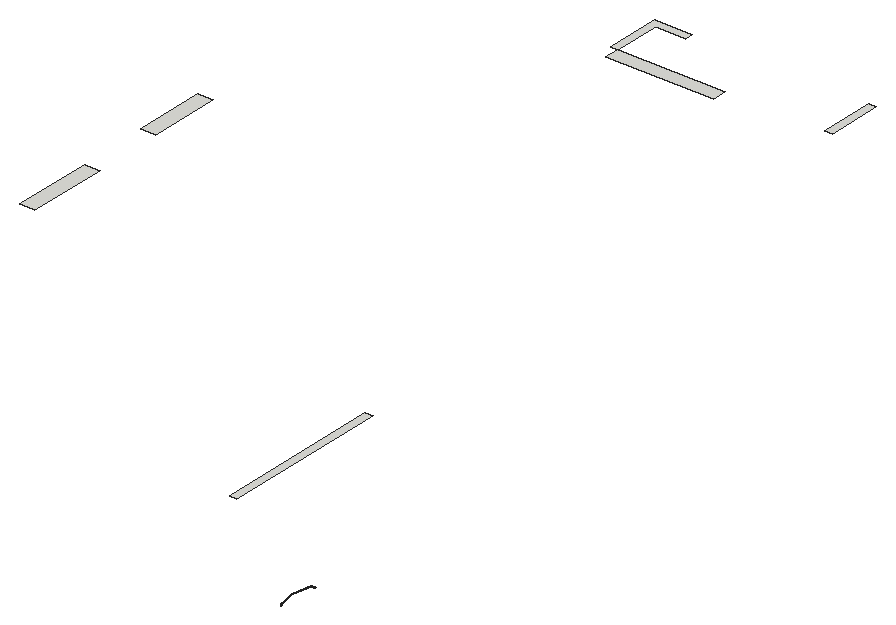
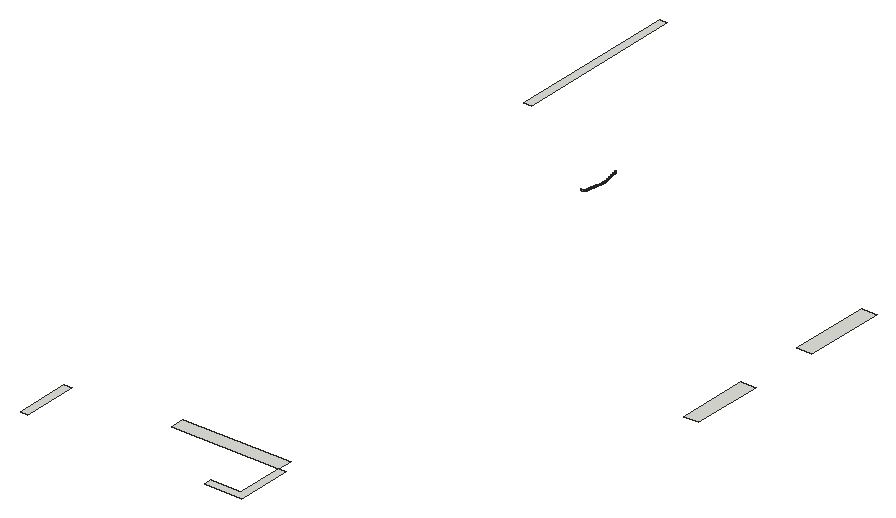
# SketchUp Ruby script. Lengths in inches.
U = 1.inch
M = Sketchup.active_model
def pt(a) = Geom::Point3d.new(a.map { |v| v * U })
def face(e, loops, mat)
  f = e.add_face(loops[0].map { |a| pt(a) })
  loops[1..].each { |l| e.add_face(l.map { |a| pt(a) }).erase! }
  f.material = f.back_material = mat if mat
  f
end
# faces: each face lists its corners as indices into pts; further lists are holes
def faces(e, pts, list, mat = nil) = list.each { |f| face(e, (f[0].is_a?(Array) ? f : [f]).map { |l| l.map { |i| pts[i] } }, mat) }
# xy, xz, yz: faces in a plane at the given z, y or x. An outline is a flat list of corners, or four numbers for a rectangle; further outlines are holes
def ring(l) = l.size == 4 ? [[l[0], l[1]], [l[2], l[1]], [l[2], l[3]], [l[0], l[3]]] : l.each_slice(2).to_a
def flat(e, list, mat, &to3) = list.each { |f| face(e, (f[0].is_a?(Array) ? f : [f]).map { |l| ring(l).map { |u, v| to3.(u, v) } }, mat) }
def xy(e, z, list, mat = nil) = flat(e, list, mat) { |x, y| [x, y, z] }
def xz(e, y, list, mat = nil) = flat(e, list, mat) { |x, z| [x, y, z] }
def yz(e, x, list, mat = nil) = flat(e, list, mat) { |y, z| [x, y, z] }
def lines(e, pts, list) = list.each { |a, b| e.add_line(pt(pts[a]), pt(pts[b])) }
# prism: a flat outline (further loops are holes) pulled along v
def prism(e, loops, v, mat = nil)
  f = face(e, loops, mat); d = Geom::Vector3d.new(v.map { |x| x * U })
  f.pushpull(f.normal.samedirection?(d) ? d.length : -d.length)
end
def box(e, o, s, mat = nil) = prism(e, [[o, [o[0] + s[0], o[1], o[2]], [o[0] + s[0], o[1] + s[1], o[2]], [o[0], o[1] + s[1], o[2]]]], [0, 0, s[2]], mat)
def at(x, y, z, deg = 0) = Geom::Transformation.translation(pt([x, y, z])) * Geom::Transformation.rotation(ORIGIN, Z_AXIS, deg.degrees)
def axes(o, x, y, z) = Geom::Transformation.new([*x, 0, *y, 0, *z, 0, *pt(o).to_a, 1])
def part(name) = M.definitions.add(name)
# library, detail: a bought-in or finely detailed component or shape, given as its bounding box
def library(name, o, s) = part(name).tap { |d| box(d.entities, o, s) }
def detail(e, o, s) = box(e.add_group.entities, o, s)
def put(e, d, t, mat = nil) = e.add_instance(d, t).tap { |i| i.material = mat if mat }
def group(e, t, mat = nil) = e.add_group.tap { |g| g.transformation = t; g.material = mat if mat }.entities
root = M.entities
xy(root,108,[[322.5,47.86,327,149.86],[71,204.86,80,253.05],[198,486.86,262.5,495.62],[193.5,495.875,198,495.875,198,524.36,216.18,524.36,216.18,528.86,193.5,528.86],[322.5,495.875,327,528.86]])
xy(root,108.57,[[71,295.7,80,338.36]])
p = [[329.39,77.66,38.26],[329.36,77.63,38.17],[329.28,77.71,38.17],[329.31,77.74,38.26],[329.48,77.59,38.26],[329.46,77.55,38.17],
  [329.2,77.8,38.17],[329.23,77.82,38.26],[329.13,77.9,38.17],[329.17,77.92,38.26],[329.08,78,38.17],[329.12,78.02,38.26],
  [329.04,78.11,38.17],[329.07,78.125,38.26],[329,78.23,38.17],[329.04,78.24,38.26],[328.96,78.42,38.17],[329,78.43,38.26],
  [328.93,78.61,38.17],[328.97,78.62,38.26],[328.9,78.81,38.17],[328.9375,78.8125,38.26],[328.87,79,38.17],[328.91,79.01,38.26],
  [328.85,79.2,38.17],[328.89,79.2,38.26],[328.83,79.39,38.17],[328.87,79.4,38.26],[328.82,79.59,38.17],[328.86,79.59,38.26],
  [328.8125,79.78,38.17],[328.85,79.79,38.26],[328.8125,79.98,38.17],[328.85,79.98,38.26],[328.8125,80.18,38.17],[328.85,80.18,38.26],
  [328.82,80.375,38.17],[328.86,80.37,38.26],[328.83,80.59,38.17],[328.875,80.59,38.26],[328.61,81.3,38.17],[328.65,81.31,38.26],
  [328.4,81.99,38.17],[328.44,82,38.26],[328.21,82.6875,38.17],[328.25,82.7,38.26],[328.03,83.39,38.17],[328.07,83.4,38.26],
  [327.87,84.09,38.17],[327.91,84.1,38.26],[327.72,84.8,38.17],[327.75,84.8125,38.26],[327.58,85.51,38.17],[327.62,85.52,38.26],
  [327.45,86.23,38.17],[327.49,86.23,38.26],[327.34,86.94,38.17],[327.38,86.95,38.26],[327.24,87.66,38.17],[327.28,87.67,38.26],
  [327.16,88.38,38.17],[327.2,88.38,38.26],[327.09,89.09,38.17],[327.13,89.09,38.26],[327.16,89.81,38.17],[327.2,89.8,38.26],
  [327.24,90.53,38.17],[327.28,90.52,38.26],[327.34,91.24,38.17],[327.38,91.24,38.26],[327.45,91.96,38.17],[327.49,91.95,38.26],
  [327.58,92.67,38.17],[327.62,92.66,38.26],[327.72,93.38,38.17],[327.75,93.375,38.26],[327.87,94.09,38.17],[327.91,94.08,38.26],
  [328.03,94.8,38.17],[328.07,94.79,38.26],[328.21,95.5,38.17],[328.25,95.49,38.26],[328.4,96.2,38.17],[328.44,96.19,38.26],
  [328.61,96.89,38.17],[328.65,96.88,38.26],[328.83,97.6,38.17],[328.875,97.59,38.26],[328.82,97.8125,38.17],[328.86,97.8125,38.26],
  [328.8125,98.01,38.17],[328.85,98.01,38.26],[328.8125,98.21,38.17],[328.85,98.21,38.26],[328.8125,98.4,38.17],[328.85,98.4,38.26],
  [328.82,98.6,38.17],[328.86,98.6,38.26],[328.83,98.79,38.17],[328.87,98.79,38.26],[328.85,98.99,38.17],[328.89,98.99,38.26],
  [328.87,99.18,38.17],[328.91,99.18,38.26],[328.9,99.38,38.17],[328.9375,99.375,38.26],[328.93,99.57,38.17],[328.97,99.57,38.26],
  [328.96,99.77,38.17],[329,99.76,38.26],[329,99.96,38.17],[329.04,99.95,38.26],[329.04,100.07,38.17],[329.07,100.06,38.26],
  [329.08,100.18,38.17],[329.12,100.17,38.26],[329.13,100.29,38.17],[329.17,100.27,38.26],[329.2,100.39,38.17],[329.23,100.36,38.26],
  [329.28,100.48,38.17],[329.31,100.45,38.26],[329.36,100.56,38.17],[329.39,100.53,38.26],[329.46,100.63,38.17],[329.48,100.6,38.26],
  [329.56,100.69,38.17],[329.58,100.66,38.26],[329.66,100.75,38.17],[329.68,100.71,38.26],[329.77,100.79,38.17],[329.79,100.75,38.26],
  [329.89,100.8125,38.17],[329.9,100.77,38.26],[330.01,100.83,38.17],[330.01,100.79,38.26],[331.77,100.9375,38.17],[331.77,100.9,38.26],
  [329.6,77.57,38.34],[329.58,77.53,38.26],[329.5,77.625,38.34],[329.72,77.57,38.42],[329.7,77.52,38.34],[329.625,77.61,38.42],
  [329.42,77.69,38.34],[329.54,77.67,38.42],[329.45,77.73,38.42],[329.34,77.77,38.34],[329.27,77.85,38.34],[329.38,77.8,38.42],
  [329.21,77.94,38.34],[329.3125,77.88,38.42],[329.16,78.04,38.34],[329.25,77.97,38.42],[329.21,78.0625,38.42],[329.12,78.14,38.34],
  [329.17,78.16,38.42],[329.09,78.25,38.34],[329.14,78.26,38.42],[329.05,78.4375,38.34],[329.1,78.45,38.42],[329.01,78.63,38.34],
  [329.07,78.64,38.42],[328.98,78.82,38.34],[329.03,78.83,38.42],[328.96,79.01,38.34],[329.01,79.02,38.42],[328.94,79.2,38.34],
  [328.99,79.21,38.42],[328.92,79.4,38.34],[328.97,79.4,38.42],[328.91,79.59,38.34],[328.96,79.59,38.42],[328.9,79.79,38.34],
  [328.95,79.79,38.42],[328.9,79.98,38.34],[328.95,79.98,38.42],[328.9,80.18,38.34],[328.95,80.17,38.42],[328.91,80.37,38.34],
  [328.96,80.37,38.42],[328.92,80.6,38.34],[328.97,80.6,38.42],[328.69,81.32,38.34],[328.74,81.34,38.42],[328.49,82.01,38.34],
  [328.54,82.03,38.42],[328.29,82.71,38.34],[328.35,82.72,38.42],[328.12,83.41,38.34],[328.17,83.42,38.42],[327.95,84.11,38.34],
  [328,84.125,38.42],[327.8,84.82,38.34],[327.85,84.83,38.42],[327.66,85.53,38.34],[327.71,85.54,38.42],[327.54,86.24,38.34],
  [327.59,86.25,38.42],[327.43,86.96,38.34],[327.48,86.96,38.42],[327.33,87.67,38.34],[327.38,87.68,38.42],[327.25,88.39,38.34],
  [327.3,88.39,38.42],[327.18,89.09,38.34],[327.23,89.09,38.42],[327.25,89.8,38.34],[327.3,89.79,38.42],[327.33,90.51,38.34],
  [327.38,90.51,38.42],[327.43,91.23,38.34],[327.48,91.22,38.42],[327.54,91.94,38.34],[327.59,91.9375,38.42],[327.66,92.66,38.34],
  [327.71,92.65,38.42],[327.8,93.37,38.34],[327.85,93.36,38.42],[327.95,94.07,38.34],[328,94.0625,38.42],[328.12,94.78,38.34],
  [328.17,94.76,38.42],[328.29,95.48,38.34],[328.35,95.46,38.42],[328.49,96.17,38.34],[328.54,96.16,38.42],[328.69,96.87,38.34],
  [328.74,96.85,38.42],[328.92,97.59,38.34],[328.97,97.58,38.42],[328.91,97.82,38.34],[328.96,97.82,38.42],[328.9,98.01,38.34],
  [328.95,98.01,38.42],[328.9,98.2,38.34],[328.95,98.2,38.42],[328.9,98.4,38.34],[328.95,98.4,38.42],[328.91,98.59,38.34],
  [328.96,98.59,38.42],[328.92,98.79,38.34],[328.97,98.78,38.42],[328.94,98.98,38.34],[328.99,98.98,38.42],[328.96,99.17,38.34],
  [329.01,99.17,38.42],[328.98,99.37,38.34],[329.03,99.36,38.42],[329.01,99.56,38.34],[329.07,99.55,38.42],[329.05,99.75,38.34],
  [329.1,99.74,38.42],[329.09,99.9375,38.34],[329.14,99.92,38.42],[329.12,100.04,38.34],[329.17,100.03,38.42],[329.16,100.15,38.34],
  [329.21,100.125,38.42],[329.21,100.24,38.34],[329.25,100.22,38.42],[329.27,100.33,38.34],[329.3125,100.3,38.42],[329.34,100.42,38.34],
  [329.38,100.38,38.42],[329.42,100.49,38.34],[329.45,100.45,38.42],[329.5,100.5625,38.34],[329.54,100.52,38.42],[329.6,100.62,38.34],
  [329.625,100.57,38.42],[329.7,100.67,38.34],[329.72,100.62,38.42],[329.8,100.7,38.34],[329.8125,100.65,38.42],[329.91,100.73,38.34],
  [329.92,100.68,38.42],[330.02,100.74,38.34],[330.02,100.69,38.42],[331.78,100.85,38.34],[329.83,77.59,38.5],[329.8125,77.53,38.42],
  [329.74,77.625,38.5],[329.93,77.57,38.5],[329.92,77.51,38.42],[329.65,77.67,38.5],[329.57,77.72,38.5],[329.49,77.78,38.5],
  [329.42,77.84,38.5],[329.36,77.92,38.5],[329.31,78,38.5],[329.26,78.09,38.5],[329.22,78.18,38.5],[329.2,78.28,38.5],
  [329.16,78.46,38.5],[329.125,78.65,38.5],[329.09,78.84,38.5],[329.07,79.03,38.5],[329.05,79.22,38.5],[329.03,79.41,38.5],
  [329.02,79.6,38.5],[329.01,79.79,38.5],[329.01,79.98,38.5],[329.01,80.17,38.5],[329.02,80.36,38.5],[329.03,80.61,38.5],
  [328.8,81.35,38.5],[328.59,82.04,38.5],[328.4,82.74,38.5],[328.22,83.4375,38.5],[328.06,84.14,38.5],[327.91,84.84,38.5],
  [327.77,85.55,38.5],[327.65,86.26,38.5],[327.54,86.97,38.5],[327.44,87.69,38.5],[327.36,88.4,38.5],[327.29,89.09,38.5],
  [327.36,89.78,38.5],[327.44,90.5,38.5],[327.54,91.21,38.5],[327.65,91.93,38.5],[327.77,92.64,38.5],[327.91,93.34,38.5],
  [328.06,94.05,38.5],[328.22,94.75,38.5],[328.4,95.45,38.5],[328.59,96.14,38.5],[328.8,96.83,38.5],[329.03,97.57,38.5],
  [329.02,97.82,38.5],[329.01,98.01,38.5],[329.01,98.2,38.5],[329.01,98.4,38.5],[329.02,98.59,38.5],[329.03,98.78,38.5],
  [329.05,98.97,38.5],[329.07,99.16,38.5],[329.09,99.35,38.5],[329.125,99.54,38.5],[329.16,99.73,38.5],[329.2,99.91,38.5],
  [329.22,100.01,38.5],[329.26,100.1,38.5],[329.31,100.1875,38.5],[329.36,100.27,38.5],[329.42,100.34,38.5],[329.49,100.41,38.5],
  [329.57,100.47,38.5],[329.65,100.52,38.5],[329.74,100.5625,38.5],[329.83,100.6,38.5],[329.93,100.62,38.5],[330.03,100.63,38.5],
  [329.85,77.65,38.57],[329.76,77.68,38.57],[329.68,77.72,38.57],[329.9375,77.63,38.57],[330.03,77.62,38.57],[330.03,77.55,38.5],
  [329.61,77.77,38.57],[329.53,77.83,38.57],[329.47,77.89,38.57],[329.41,77.96,38.57],[329.36,78.03,38.57],[329.32,78.11,38.57],
  [329.29,78.2,38.57],[329.26,78.29,38.57],[329.22,78.47,38.57],[329.1875,78.66,38.57],[329.16,78.84,38.57],[329.13,79.03,38.57],
  [329.11,79.22,38.57],[329.09,79.41,38.57],[329.08,79.6,38.57],[329.08,79.79,38.57],[329.07,79.98,38.57],[329.08,80.17,38.57],
  [329.08,80.36,38.57],[329.1,80.62,38.57],[328.86,81.37,38.57],[328.66,82.0625,38.57],[328.47,82.76,38.57],[328.29,83.45,38.57],
  [328.125,84.15,38.57],[327.97,84.86,38.57],[327.84,85.5625,38.57],[327.71,86.27,38.57],[327.6,86.98,38.57],[327.51,87.69,38.57],
  [327.42,88.41,38.57],[327.36,89.09,38.57],[327.42,89.78,38.57],[327.51,90.49,38.57],[327.6,91.21,38.57],[327.71,91.92,38.57],
  [327.84,92.625,38.57],[327.97,93.33,38.57],[328.125,94.03,38.57],[328.29,94.73,38.57],[328.47,95.43,38.57],[328.66,96.125,38.57],
  [328.86,96.8125,38.57],[329.1,97.57,38.57],[329.08,97.83,38.57],[329.08,98.01,38.57],[329.07,98.2,38.57],[329.08,98.39,38.57],
  [329.08,98.58,38.57],[329.09,98.77,38.57],[329.11,98.96,38.57],[329.13,99.15,38.57],[329.16,99.34,38.57],[329.1875,99.53,38.57],
  [329.22,99.72,38.57],[329.26,99.89,38.57],[329.29,99.99,38.57],[329.32,100.07,38.57],[329.36,100.15,38.57],[329.41,100.23,38.57],
  [329.47,100.3,38.57],[329.53,100.36,38.57],[329.61,100.42,38.57],[329.68,100.46,38.57],[329.76,100.5,38.57],[329.85,100.53,38.57],
  [329.9375,100.55,38.57],[330.03,100.57,38.57],[329.95,77.7,38.64],[329.87,77.72,38.64],[330.04,77.6875,38.64],[329.72,77.78,38.64],
  [329.65,77.83,38.64],[329.79,77.75,38.64],[329.82,77.82,38.7],[329.75,77.85,38.7],[329.89,77.79,38.7],[329.96,77.77,38.7],
  [330.05,77.76,38.7],[329.58,77.88,38.64],[329.52,77.9375,38.64],[329.6875,77.89,38.7],[329.63,77.94,38.7],[329.47,78,38.64],
  [329.58,77.99,38.7],[329.53,78.05,38.7],[329.42,78.07,38.64],[329.38,78.14,38.64],[329.49,78.11,38.7],[329.35,78.22,38.64],
  [329.45,78.17,38.7],[329.42,78.24,38.7],[329.33,78.31,38.64],[329.4,78.33,38.7],[329.29,78.48,38.64],[329.36,78.5,38.7],
  [329.26,78.67,38.64],[329.33,78.68,38.7],[329.23,78.86,38.64],[329.3,78.87,38.7],[329.2,79.04,38.64],[329.28,79.05,38.7],
  [329.18,79.23,38.64],[329.25,79.24,38.7],[329.16,79.42,38.64],[329.24,79.42,38.7],[329.15,79.6,38.64],[329.23,79.61,38.7],
  [329.15,79.79,38.64],[329.22,79.79,38.7],[329.14,79.98,38.64],[329.22,79.98,38.7],[329.15,80.17,38.64],[329.22,80.17,38.7],
  [329.15,80.36,38.64],[329.23,80.35,38.7],[329.17,80.63,38.64],[329.24,80.64,38.7],[328.93,81.39,38.64],[329,81.41,38.7],
  [328.72,82.08,38.64],[328.8,82.1,38.7],[328.53,82.77,38.64],[328.61,82.79,38.7],[328.36,83.47,38.64],[328.43,83.49,38.7],
  [328.19,84.17,38.64],[328.26,84.18,38.7],[328.04,84.87,38.64],[328.11,84.88,38.7],[327.9,85.57,38.64],[327.98,85.59,38.7],
  [327.78,86.28,38.64],[327.85,86.29,38.7],[327.67,86.99,38.64],[327.75,87,38.7],[327.57,87.7,38.64],[327.65,87.71,38.7],
  [327.49,88.42,38.64],[327.57,88.42,38.7],[327.43,89.09,38.64],[327.5,89.09,38.7],[327.49,89.77,38.64],[327.57,89.76,38.7],
  [327.57,90.48,38.64],[327.65,90.47,38.7],[327.67,91.2,38.64],[327.75,91.18,38.7],[327.78,91.9,38.64],[327.85,91.89,38.7],
  [327.9,92.61,38.64],[327.98,92.6,38.7],[328.04,93.32,38.64],[328.11,93.3,38.7],[328.19,94.02,38.64],[328.26,94,38.7],
  [328.36,94.72,38.64],[328.43,94.7,38.7],[328.53,95.41,38.64],[328.61,95.39,38.7],[328.72,96.1,38.64],[328.8,96.08,38.7],
  [328.93,96.79,38.64],[329,96.77,38.7],[329.17,97.56,38.64],[329.24,97.55,38.7],[329.15,97.83,38.64],[329.23,97.83,38.7],
  [329.15,98.02,38.64],[329.22,98.02,38.7],[329.14,98.2,38.64],[329.22,98.2,38.7],[329.15,98.39,38.64],[329.22,98.39,38.7],
  [329.15,98.58,38.64],[329.23,98.58,38.7],[329.16,98.77,38.64],[329.24,98.76,38.7],[329.18,98.96,38.64],[329.25,98.95,38.7],
  [329.2,99.14,38.64],[329.28,99.13,38.7],[329.23,99.33,38.64],[329.3,99.32,38.7],[329.26,99.52,38.64],[329.33,99.5,38.7],
  [329.29,99.7,38.64],[329.36,99.6875,38.7],[329.33,99.88,38.64],[329.4,99.86,38.7],[329.35,99.97,38.64],[329.42,99.94,38.7],
  [329.38,100.04,38.64],[329.45,100.01,38.7],[329.42,100.12,38.64],[329.49,100.08,38.7],[329.47,100.1875,38.64],[329.53,100.14,38.7],
  [329.52,100.25,38.64],[329.58,100.2,38.7],[329.58,100.31,38.64],[329.63,100.25,38.7],[329.65,100.36,38.64],[329.6875,100.3,38.7],
  [329.72,100.4,38.64],[329.75,100.34,38.7],[329.79,100.4375,38.64],[329.82,100.37,38.7],[329.87,100.47,38.64],[329.89,100.39,38.7],
  [329.95,100.49,38.64],[329.96,100.41,38.7],[330.04,100.5,38.64],[330.05,100.42,38.7],[61.5,107.65,72],[52.7,107.65,72],
  [216.125,495.62,71.875],[216.125,495.62,72]]
faces(root,p,[[0,1,2,3],[4,5,1,0],[3,2,6,7],[7,6,8,9],[9,8,10,11],[11,10,12,13],[13,12,14,15],[15,14,16,17],
  [17,16,18,19],[19,18,20,21],[21,20,22,23],[23,22,24,25],[25,24,26,27],[27,26,28,29],[29,28,30,31],[31,30,32,33],
  [33,32,34,35],[35,34,36,37],[37,36,38,39],[39,38,40,41],[41,40,42,43],[43,42,44,45],[45,44,46,47],[47,46,48,49],
  [49,48,50,51],[51,50,52,53],[53,52,54,55],[55,54,56,57],[57,56,58,59],[59,58,60,61],[61,60,62,63],[63,62,64,65],
  [65,64,66,67],[67,66,68,69],[69,68,70,71],[71,70,72,73],[73,72,74,75],[75,74,76,77],[77,76,78,79],[79,78,80,81],
  [81,80,82,83],[83,82,84,85],[85,84,86,87],[87,86,88,89],[89,88,90,91],[91,90,92,93],[93,92,94,95],[95,94,96,97],
  [97,96,98,99],[99,98,100,101],[101,100,102,103],[103,102,104,105],[105,104,106,107],[107,106,108,109],[109,108,110,111],[111,110,112,113],
  [113,112,114,115],[115,114,116,117],[117,116,118,119],[119,118,120,121],[121,120,122,123],[123,122,124,125],[125,124,126,127],[127,126,128,129],
  [129,128,130,131],[131,130,132,133],[133,132,134,135],[135,134,136,137],[138,139,4,140],[141,142,138,143],[140,4,0,144],[145,140,144,146],
  [143,138,140,145],[147,3,7,148],[144,0,3,147],[146,144,147,149],[148,7,9,150],[149,147,148,151],[150,9,11,152],[151,148,150,153],
  [153,150,152,154],[152,11,13,155],[154,152,155,156],[155,13,15,157],[156,155,157,158],[157,15,17,159],[158,157,159,160],[159,17,19,161],
  [160,159,161,162],[161,19,21,163],[162,161,163,164],[163,21,23,165],[164,163,165,166],[165,23,25,167],[166,165,167,168],[167,25,27,169],
  [168,167,169,170],[169,27,29,171],[170,169,171,172],[171,29,31,173],[172,171,173,174],[173,31,33,175],[174,173,175,176],[176,175,177,178],
  [175,33,35,177],[178,177,179,180],[177,35,37,179],[179,37,39,181],[180,179,181,182],[181,39,41,183],[182,181,183,184],[183,41,43,185],
  [184,183,185,186],[185,43,45,187],[186,185,187,188],[187,45,47,189],[188,187,189,190],[189,47,49,191],[190,189,191,192],[191,49,51,193],
  [192,191,193,194],[193,51,53,195],[194,193,195,196],[195,53,55,197],[196,195,197,198],[197,55,57,199],[198,197,199,200],[199,57,59,201],
  [200,199,201,202],[201,59,61,203],[202,201,203,204],[203,61,63,205],[204,203,205,206],[205,63,65,207],[206,205,207,208],[208,207,209,210],
  [207,65,67,209],[210,209,211,212],[209,67,69,211],[212,211,213,214],[211,69,71,213],[214,213,215,216],[213,71,73,215],[216,215,217,218],
  [215,73,75,217],[218,217,219,220],[217,75,77,219],[219,77,79,221],[220,219,221,222],[222,221,223,224],[221,79,81,223],[223,81,83,225],
  [224,223,225,226],[225,83,85,227],[226,225,227,228],[228,227,229,230],[227,85,87,229],[230,229,231,232],[229,87,89,231],[231,89,91,233],
  [232,231,233,234],[233,91,93,235],[234,233,235,236],[236,235,237,238],[235,93,95,237],[238,237,239,240],[237,95,97,239],[240,239,241,242],
  [239,97,99,241],[242,241,243,244],[241,99,101,243],[244,243,245,246],[243,101,103,245],[245,103,105,247],[246,245,247,248],[247,105,107,249],
  [248,247,249,250],[250,249,251,252],[249,107,109,251],[252,251,253,254],[251,109,111,253],[253,111,113,255],[254,253,255,256],[256,255,257,258],
  [255,113,115,257],[257,115,117,259],[258,257,259,260],[260,259,261,262],[259,117,119,261],[261,119,121,263],[262,261,263,264],[264,263,265,266],
  [263,121,123,265],[266,265,267,268],[265,123,125,267],[268,267,269,270],[267,125,127,269],[270,269,271,272],[269,127,129,271],[272,271,273,274],
  [271,129,131,273],[274,273,275,276],[273,131,133,275],[276,275,277,278],[275,133,135,277],[277,135,137,279],[280,281,141,282],[283,284,281,280],
  [285,143,145,286],[282,141,143,285],[287,146,149,288],[286,145,146,287],[288,149,151,289],[289,151,153,290],[290,153,154,291],[291,154,156,292],
  [292,156,158,293],[293,158,160,294],[294,160,162,295],[295,162,164,296],[296,164,166,297],[297,166,168,298],[298,168,170,299],[299,170,172,300],
  [300,172,174,301],[301,174,176,302],[302,176,178,303],[303,178,180,304],[304,180,182,305],[305,182,184,306],[306,184,186,307],[307,186,188,308],
  [308,188,190,309],[309,190,192,310],[310,192,194,311],[311,194,196,312],[312,196,198,313],[313,198,200,314],[314,200,202,315],[315,202,204,316],
  [316,204,206,317],[317,206,208,318],[318,208,210,319],[319,210,212,320],[320,212,214,321],[321,214,216,322],[322,216,218,323],[323,218,220,324],
  [324,220,222,325],[325,222,224,326],[326,224,226,327],[327,226,228,328],[328,228,230,329],[329,230,232,330],[330,232,234,331],[331,234,236,332],
  [332,236,238,333],[333,238,240,334],[334,240,242,335],[335,242,244,336],[336,244,246,337],[337,246,248,338],[338,248,250,339],[339,250,252,340],
  [340,252,254,341],[341,254,256,342],[342,256,258,343],[343,258,260,344],[344,260,262,345],[345,262,264,346],[346,264,266,347],[347,266,268,348],
  [348,268,270,349],[349,270,272,350],[350,272,274,351],[351,274,276,352],[352,276,278,353],[354,280,282,355],[355,282,285,356],[357,283,280,354],
  [358,359,283,357],[360,286,287,361],[356,285,286,360],[361,287,288,362],[362,288,289,363],[363,289,290,364],[364,290,291,365],[365,291,292,366],
  [366,292,293,367],[367,293,294,368],[368,294,295,369],[369,295,296,370],[370,296,297,371],[371,297,298,372],[372,298,299,373],[373,299,300,374],
  [374,300,301,375],[375,301,302,376],[376,302,303,377],[377,303,304,378],[378,304,305,379],[379,305,306,380],[380,306,307,381],[381,307,308,382],
  [382,308,309,383],[383,309,310,384],[384,310,311,385],[385,311,312,386],[386,312,313,387],[387,313,314,388],[388,314,315,389],[389,315,316,390],
  [390,316,317,391],[391,317,318,392],[392,318,319,393],[393,319,320,394],[394,320,321,395],[395,321,322,396],[396,322,323,397],[397,323,324,398],
  [398,324,325,399],[399,325,326,400],[400,326,327,401],[401,327,328,402],[402,328,329,403],[403,329,330,404],[404,330,331,405],[405,331,332,406],
  [406,332,333,407],[407,333,334,408],[408,334,335,409],[409,335,336,410],[410,336,337,411],[411,337,338,412],[412,338,339,413],[413,339,340,414],
  [414,340,341,415],[415,341,342,416],[416,342,343,417],[417,343,344,418],[418,344,345,419],[419,345,346,420],[420,346,347,421],[421,347,348,422],
  [422,348,349,423],[423,349,350,424],[424,350,351,425],[425,351,352,426],[426,352,353,427],[428,357,354,429],[430,358,357,428],[431,356,360,432],
  [433,355,356,431],[434,433,431,435],[429,354,355,433],[436,429,433,434],[437,428,429,436],[438,430,428,437],[432,360,361,439],[439,361,362,440],
  [435,431,432,441],[441,432,439,442],[440,362,363,443],[442,439,440,444],[444,440,443,445],[446,364,365,447],[443,363,364,446],[445,443,446,448],
  [447,365,366,449],[448,446,447,450],[450,447,449,451],[449,366,367,452],[451,449,452,453],[452,367,368,454],[453,452,454,455],[454,368,369,456],
  [455,454,456,457],[456,369,370,458],[457,456,458,459],[458,370,371,460],[459,458,460,461],[460,371,372,462],[461,460,462,463],[462,372,373,464],
  [463,462,464,465],[464,373,374,466],[465,464,466,467],[466,374,375,468],[467,466,468,469],[468,375,376,470],[469,468,470,471],[471,470,472,473],
  [470,376,377,472],[473,472,474,475],[472,377,378,474],[474,378,379,476],[475,474,476,477],[476,379,380,478],[477,476,478,479],[478,380,381,480],
  [479,478,480,481],[480,381,382,482],[481,480,482,483],[482,382,383,484],[483,482,484,485],[484,383,384,486],[485,484,486,487],[486,384,385,488],
  [487,486,488,489],[488,385,386,490],[489,488,490,491],[490,386,387,492],[491,490,492,493],[492,387,388,494],[493,492,494,495],[494,388,389,496],
  [495,494,496,497],[496,389,390,498],[497,496,498,499],[498,390,391,500],[499,498,500,501],[501,500,502,503],[500,391,392,502],[502,392,393,504],
  [503,502,504,505],[504,393,394,506],[505,504,506,507],[506,394,395,508],[507,506,508,509],[508,395,396,510],[509,508,510,511],[510,396,397,512],
  [511,510,512,513],[513,512,514,515],[512,397,398,514],[514,398,399,516],[515,514,516,517],[516,399,400,518],[517,516,518,519],[519,518,520,521],
  [518,400,401,520],[521,520,522,523],[520,401,402,522],[523,522,524,525],[522,402,403,524],[525,524,526,527],[524,403,404,526],[526,404,405,528],
  [527,526,528,529],[528,405,406,530],[529,528,530,531],[531,530,532,533],[530,406,407,532],[533,532,534,535],[532,407,408,534],[534,408,409,536],
  [535,534,536,537],[536,409,410,538],[537,536,538,539],[539,538,540,541],[538,410,411,540],[540,411,412,542],[541,540,542,543],[543,542,544,545],
  [542,412,413,544],[544,413,414,546],[545,544,546,547],[546,414,415,548],[547,546,548,549],[549,548,550,551],[548,415,416,550],[551,550,552,553],
  [550,416,417,552],[552,417,418,554],[553,552,554,555],[555,554,556,557],[554,418,419,556],[557,556,558,559],[556,419,420,558],[559,558,560,561],
  [558,420,421,560],[560,421,422,562],[561,560,562,563],[563,562,564,565],[565,564,566,567],[562,422,423,564],[564,423,424,566],[567,566,568,569],
  [566,424,425,568],[569,568,570,571],[571,570,572,573],[568,425,426,570],[570,426,427,572]])
lines(root,p,[[574,575],[576,577]])
